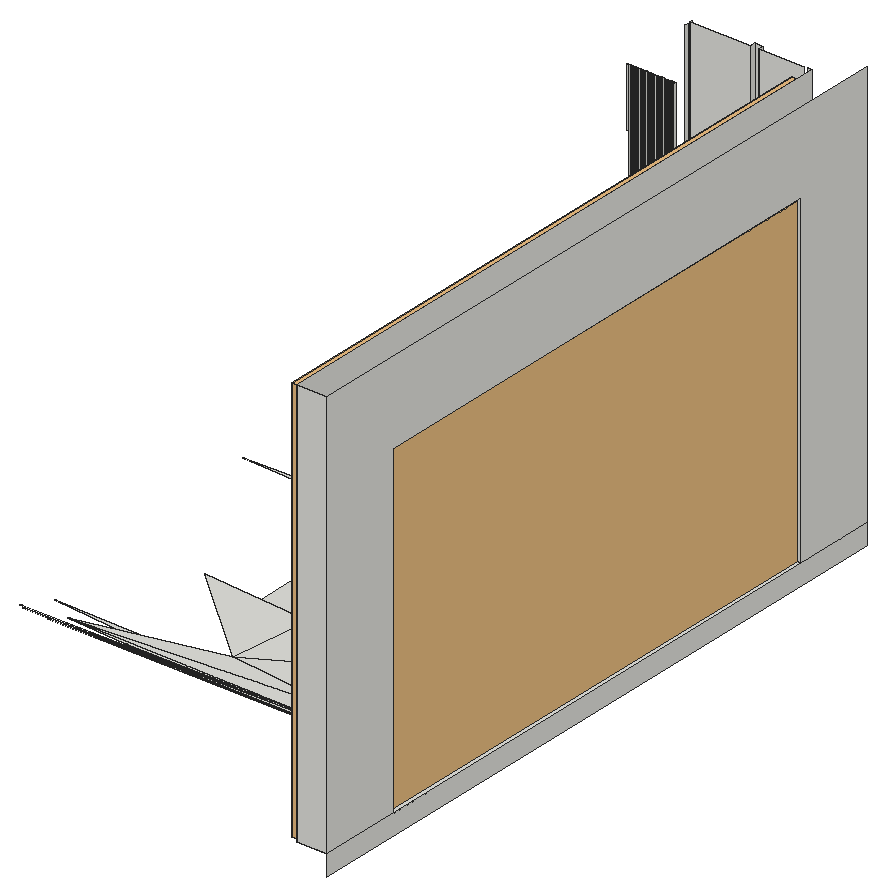
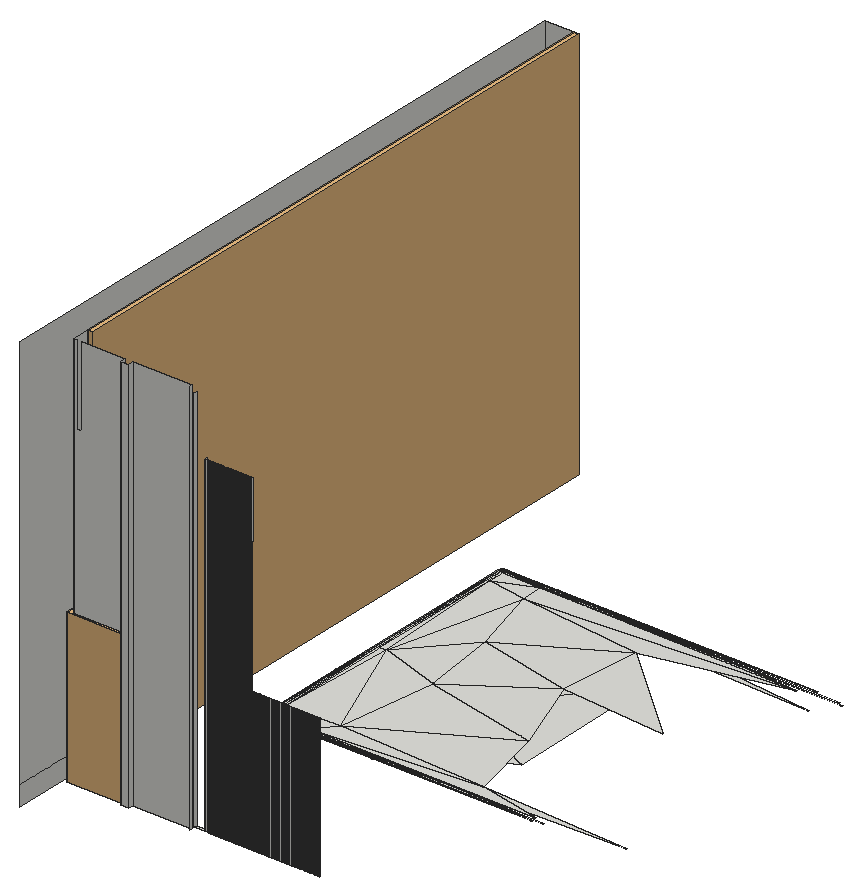
# SketchUp Ruby script. Lengths in inches.
U = 1.inch
M = Sketchup.active_model
def pt(a) = Geom::Point3d.new(a.map { |v| v * U })
def face(e, loops, mat)
  f = e.add_face(loops[0].map { |a| pt(a) })
  loops[1..].each { |l| e.add_face(l.map { |a| pt(a) }).erase! }
  f.material = f.back_material = mat if mat
  f
end
# faces: each face lists its corners as indices into pts; further lists are holes
def faces(e, pts, list, mat = nil) = list.each { |f| face(e, (f[0].is_a?(Array) ? f : [f]).map { |l| l.map { |i| pts[i] } }, mat) }
# xy, xz, yz: faces in a plane at the given z, y or x. An outline is a flat list of corners, or four numbers for a rectangle; further outlines are holes
def ring(l) = l.size == 4 ? [[l[0], l[1]], [l[2], l[1]], [l[2], l[3]], [l[0], l[3]]] : l.each_slice(2).to_a
def flat(e, list, mat, &to3) = list.each { |f| face(e, (f[0].is_a?(Array) ? f : [f]).map { |l| ring(l).map { |u, v| to3.(u, v) } }, mat) }
def xy(e, z, list, mat = nil) = flat(e, list, mat) { |x, y| [x, y, z] }
def xz(e, y, list, mat = nil) = flat(e, list, mat) { |x, z| [x, y, z] }
def yz(e, x, list, mat = nil) = flat(e, list, mat) { |y, z| [x, y, z] }
def lines(e, pts, list) = list.each { |a, b| e.add_line(pt(pts[a]), pt(pts[b])) }
# prism: a flat outline (further loops are holes) pulled along v
def prism(e, loops, v, mat = nil)
  f = face(e, loops, mat); d = Geom::Vector3d.new(v.map { |x| x * U })
  f.pushpull(f.normal.samedirection?(d) ? d.length : -d.length)
end
def box(e, o, s, mat = nil) = prism(e, [[o, [o[0] + s[0], o[1], o[2]], [o[0] + s[0], o[1] + s[1], o[2]], [o[0], o[1] + s[1], o[2]]]], [0, 0, s[2]], mat)
def at(x, y, z, deg = 0) = Geom::Transformation.translation(pt([x, y, z])) * Geom::Transformation.rotation(ORIGIN, Z_AXIS, deg.degrees)
def axes(o, x, y, z) = Geom::Transformation.new([*x, 0, *y, 0, *z, 0, *pt(o).to_a, 1])
def part(name) = M.definitions.add(name)
# library, detail: a bought-in or finely detailed component or shape, given as its bounding box
def library(name, o, s) = part(name).tap { |d| box(d.entities, o, s) }
def detail(e, o, s) = box(e.add_group.entities, o, s)
def put(e, d, t, mat = nil) = e.add_instance(d, t).tap { |i| i.material = mat if mat }
def group(e, t, mat = nil) = e.add_group.tap { |g| g.transformation = t; g.material = mat if mat }.entities
root = M.entities
c1 = library("Potted Plant 60-25",[-10.7,-10.47,0],[21.2,21.27,47.12])
c2 = library("Curtains 001",[-91.88,-6.87,0.16],[183.71,15.03,109.46])
c3 = library("Window 46-47",[-61.02,-2.17,0],[122.04,4.34,74.02])
xy(root,0,[[189,0,198,24],[189,24,198,174],[79.4375,45.79,129.55,46.18,156.43,45.79],[156.43,45.79,129.55,46.18,161.8,46.18],[156.43,45.79,161.8,46.18,172.9375,45.79],
  [172.9375,45.79,161.8,46.18,172.63,46.18],[172.9375,45.79,172.63,46.18,173.24,46.18],[172.9375,45.79,173.24,46.18,173.85,45.82],[173.85,45.82,173.24,46.18,173.85,46.18],[173.85,45.82,173.85,46.18,174.1875,45.84],
  [174.1875,45.84,173.85,46.18,174.21,46.18],[71.8,46.18,142.125,46.79,129.55,46.18],[129.55,46.18,142.125,46.79,161.8,46.18],[161.8,46.18,142.125,46.79,172.63,46.79],[161.8,46.18,172.63,46.79,172.63,46.18],
  [172.63,46.18,172.63,46.79,173.24,46.18],[173.24,46.18,172.63,46.79,173.24,46.79],[173.24,46.18,173.24,46.79,173.85,46.18],[173.85,46.18,173.24,46.79,173.85,46.79],[173.85,46.18,173.85,46.79,174.21,46.18],
  [174.21,46.18,173.85,46.79,174.25,47.09],[70.45,46.79,143.14,47.4,142.125,46.79],[142.125,46.79,143.14,47.4,172.63,46.79],[172.63,46.79,143.14,47.4,172.63,47.97],[172.63,46.79,172.63,47.97,173.24,47.4],
  [172.63,46.79,173.24,47.4,173.24,46.79],[173.24,46.79,173.24,47.4,173.85,46.79],[173.85,46.79,173.24,47.4,173.85,47.4],[173.85,46.79,173.85,47.4,174.25,47.09],[174.25,47.09,173.85,47.4,173.85,59.65],
  [174.25,47.09,173.85,59.65,174.25,74.37],[143.14,47.4,75.08,53.77,149.74,51.96],[143.14,47.4,149.74,51.96,172.63,47.97],[173.24,47.4,172.63,47.97,173.24,94.83],[173.24,47.4,173.24,94.83,173.85,59.65],
  [173.24,47.4,173.85,59.65,173.85,47.4],[172.63,47.97,149.74,51.96,169.97,85.51],[172.63,47.97,169.97,85.51,172.63,84.58],[172.63,47.97,172.63,84.58,173.24,94.83],[149.74,51.96,112.4,68.43,138.46,72.11],
  [149.74,51.96,138.46,72.11,169.97,85.51],[173.85,59.65,173.24,94.83,173.85,111.88],[173.85,59.65,173.85,111.88,174.25,74.37],[112.4,68.43,111.5,116.5625,139.8,102.6],[112.4,68.43,139.8,102.6,138.46,72.11],
  [138.46,72.11,139.8,102.6,158.95,87.44],[138.46,72.11,158.95,87.44,169.97,85.51],[174.25,74.37,173.85,111.88,174.25,122.24],[172.63,84.58,169.97,85.51,170.01,129.8],[172.63,84.58,170.01,129.8,172.63,133.19],
  [172.63,84.58,172.63,133.19,173.24,94.83],[169.97,85.51,139.65,129.14,170.01,129.8],[169.97,85.51,139.8,102.6,139.65,129.14],[169.97,85.51,158.95,87.44,139.8,102.6],[173.24,94.83,172.63,133.19,173.24,134.57],
  [173.24,94.83,173.24,134.57,173.85,111.88],[139.8,102.6,111.5,116.5625,139.65,129.14],[173.85,111.88,173.24,134.57,173.85,134.57],[173.85,111.88,173.85,134.57,174.25,122.24],[174.25,122.24,173.85,134.57,174.25,134.87],
  [139.65,129.14,67.21,132.46,139.03,134.57],[139.65,129.14,139.03,134.57,170.01,129.8],[170.01,129.8,139.03,134.57,172.63,134.57],[170.01,129.8,172.63,134.57,172.63,133.19],[172.63,133.19,172.63,134.57,173.24,134.57],
  [139.03,134.57,110.28,135.18,156.43,135.18],[139.03,134.57,156.43,135.18,172.63,134.57],[172.63,134.57,156.43,135.18,172.63,135.18],[172.63,134.57,172.63,135.18,173.24,134.57],[173.24,134.57,172.63,135.18,173.24,135.18],
  [173.24,134.57,173.24,135.18,173.85,134.57],[173.85,134.57,173.24,135.18,173.85,135.18],[173.85,134.57,173.85,135.18,174.25,134.87],[174.25,134.87,173.85,135.18,174.21,135.79],[110.28,135.18,92.94,135.79,145.92,135.79],
  [110.28,135.18,145.92,135.79,156.43,135.18],[156.43,135.18,145.92,135.79,168.42,135.79],[156.43,135.18,168.42,135.79,172.63,135.18],[172.63,135.18,168.42,135.79,172.63,135.79],[172.63,135.18,172.63,135.79,173.24,135.18],
  [173.24,135.18,172.63,135.79,173.24,135.79],[173.24,135.18,173.24,135.79,173.85,135.18],[173.85,135.18,173.24,135.79,173.85,135.79],[173.85,135.18,173.85,135.79,174.21,135.79],[92.94,135.79,140.64,136.17,145.92,135.79],
  [145.92,135.79,140.64,136.17,168.42,135.79],[168.42,135.79,140.64,136.17,172.63,136.17],[168.42,135.79,172.63,136.17,172.63,135.79],[172.63,135.79,172.63,136.17,173.24,135.79],[173.24,135.79,172.63,136.17,173.24,136.17],
  [173.24,135.79,173.24,136.17,173.85,136.14],[173.24,135.79,173.85,136.14,173.85,135.79],[173.85,135.79,173.85,136.14,174.21,135.79],[171.08,189,173.42,190.5]])
xy(root,0.23,[[157.71,45.79,158.28,46.18,96.94,46.18],[157.71,45.79,172.9375,45.79,158.28,46.18],[172.9375,45.79,172.63,46.18,158.28,46.18],[172.9375,45.79,173.24,46.18,172.63,46.18],[172.9375,45.79,173.85,45.82,173.24,46.18],
  [173.85,45.82,173.85,46.18,173.24,46.18],[173.85,45.82,174.21,46.18,173.85,46.18],[96.94,46.18,158.28,46.18,150.44,46.79],[158.28,46.18,172.63,46.79,150.44,46.79],[158.28,46.18,172.63,46.18,172.63,46.79],
  [172.63,46.18,173.24,46.18,173.24,46.79],[172.63,46.18,173.24,46.79,172.63,46.79],[173.24,46.18,173.85,46.18,173.85,46.79],[173.24,46.18,173.85,46.79,173.24,46.79],[173.85,46.18,174.21,46.18,173.85,46.79],
  [174.21,46.18,174.25,47.09,173.85,46.79],[150.44,46.79,161.16,47.4,101.08,47.4],[150.44,46.79,172.63,46.79,161.16,47.4],[172.63,46.79,172.63,47.4,161.16,47.4],[172.63,46.79,173.24,46.79,173.24,47.4],
  [172.63,46.79,173.24,47.4,172.63,47.4],[173.24,46.79,173.85,46.79,173.85,47.4],[173.24,46.79,173.85,47.4,173.24,47.4],[173.85,46.79,174.25,47.09,173.85,47.4],[174.25,47.09,173.85,61.21,173.85,47.4],
  [174.25,47.09,174.25,62.35,173.85,61.21],[101.08,47.4,161.16,47.4,82.99,48.58],[161.16,47.4,161,54.02,82.99,48.58],[161.16,47.4,172.63,52.46,161,54.02],[161.16,47.4,172.63,47.4,172.63,52.46],
  [172.63,47.4,173.24,47.4,172.63,52.46],[173.24,47.4,173.24,85.125,172.63,52.46],[173.24,47.4,173.85,47.4,173.85,61.21],[173.24,47.4,173.85,61.21,173.24,85.125],[82.99,48.58,161,54.02,124,57.84],
  [172.63,52.46,170.8,93.47,161,54.02],[172.63,52.46,172.63,93.73,170.8,93.47],[172.63,52.46,173.24,85.125,172.63,93.73],[161,54.02,155.14,75.83,124,57.84],[161,54.02,170.8,93.47,155.14,75.83],
  [124,57.84,126.68,81.95,94.82,84.31],[124,57.84,155.14,75.83,126.68,81.95],[173.85,61.21,173.85,111.56,173.24,85.125],[173.85,61.21,174.25,62.35,173.85,111.56],[174.25,62.35,174.25,108.12,173.85,111.56],
  [155.14,75.83,152.13,99.47,126.68,81.95],[155.14,75.83,170.8,93.47,152.13,99.47],[126.68,81.95,152.13,99.47,117.31,106.81],[173.24,85.125,172.63,129.16,172.63,93.73],[173.24,85.125,173.24,134.57,172.63,129.16],
  [173.24,85.125,173.85,111.56,173.24,134.57],[170.8,93.47,156.54,128.69,152.13,99.47],[170.8,93.47,172.63,129.16,156.54,128.69],[170.8,93.47,172.63,93.73,172.63,129.16],[152.13,99.47,156.54,128.69,117.31,106.81],
  [117.31,106.81,156.54,128.69,111.91,130.52],[174.25,108.12,174.25,134.87,173.85,111.56],[173.85,111.56,173.85,134.57,173.24,134.57],[173.85,111.56,174.25,134.87,173.85,134.57],[156.54,128.69,161.15,134.57,111.91,130.52],
  [156.54,128.69,172.63,129.16,161.15,134.57],[172.63,129.16,172.63,134.57,161.15,134.57],[172.63,129.16,173.24,134.57,172.63,134.57],[111.91,130.52,161.15,134.57,92.98,134.57],[92.98,134.57,161.15,134.57,121.1,135.18],
  [161.15,134.57,162.79,135.18,121.1,135.18],[161.15,134.57,172.63,134.57,162.79,135.18],[172.63,134.57,172.63,135.18,162.79,135.18],[172.63,134.57,173.24,134.57,173.24,135.18],[172.63,134.57,173.24,135.18,172.63,135.18],
  [173.24,134.57,173.85,134.57,173.85,135.18],[173.24,134.57,173.85,135.18,173.24,135.18],[173.85,134.57,174.25,134.87,173.85,135.18],[174.25,134.87,174.21,135.79,173.85,135.18],[121.1,135.18,134.45,135.79,89.4,135.79],
  [121.1,135.18,162.6875,135.78,134.45,135.79],[121.1,135.18,162.79,135.18,162.6875,135.78],[162.79,135.18,172.63,135.79,162.6875,135.78],[162.79,135.18,172.63,135.18,172.63,135.79],[172.63,135.18,173.24,135.18,173.24,135.79],
  [172.63,135.18,173.24,135.79,172.63,135.79],[173.24,135.18,173.85,135.18,173.85,135.79],[173.24,135.18,173.85,135.79,173.24,135.79],[173.85,135.18,174.21,135.79,173.85,135.79],[162.6875,135.78,156.13,136.17,134.45,135.79],
  [162.6875,135.78,172.9375,136.17,156.13,136.17],[162.6875,135.78,172.63,135.79,172.9375,136.17],[134.45,135.79,156.13,136.17,115.29,136.17],[172.63,135.79,173.24,135.79,172.9375,136.17],[173.24,135.79,173.85,136.14,172.9375,136.17],
  [173.24,135.79,173.85,135.79,173.85,136.14],[173.85,135.79,174.1875,136.125,173.85,136.14],[173.85,135.79,174.21,135.79,174.1875,136.125]])
xy(root,1.3,[[148.625,189,151.87,189.875],[134.28,189.625,134.875,189.875],[124.28,189.75,124.875,189.875],[125.28,189.75,125.875,189.875],[126.28,189.75,126.875,189.875],
  [127.28,189.75,127.875,189.875],[128.28,189.75,128.875,189.875],[129.28,189.75,129.875,189.875],[130.28,189.75,130.875,189.875],[131.28,189.75,131.875,189.875],
  [132.28,189.75,132.875,189.875],[133.28,189.75,133.875,189.875],[135.28,189.75,135.875,189.875],[136.28,189.75,136.875,189.875],[137.28,189.75,137.875,189.875],
  [138.28,189.75,138.875,189.875],[139.28,189.75,139.875,189.875],[140.28,189.75,140.875,189.875],[141.28,189.75,141.875,189.875],[142.28,189.75,142.875,189.875],
  [143.28,189.75,143.875,189.875],[144.28,189.75,144.875,189.875],[145.28,189.75,145.875,189.875],[146.28,189.75,146.875,189.875],[147.28,189.75,147.875,189.875],
  [114.28,189.8125,114.875,189.875],[115.28,189.8125,115.875,189.875],[116.28,189.8125,116.875,189.875],[117.28,189.8125,117.875,189.875],[118.28,189.8125,118.875,189.875],
  [119.28,189.8125,119.875,189.875],[120.28,189.8125,120.875,189.875],[121.28,189.8125,121.875,189.875],[122.28,189.8125,122.875,189.875],[123.28,189.8125,123.875,189.875]])
xz(root,0,[[189,0,198,120]])
xz(root,24,[[189,0,198,96]])
xz(root,45.79,[[156.43,0,157.71,0.23,78.85,0.23],[156.43,0,172.9375,0,157.71,0.23],[172.9375,0,172.9375,0.23,157.71,0.23]])
xz(root,136.17,[[140.64,0,115.29,0.23,156.13,0.23],[140.64,0,156.13,0.23,172.63,0],[172.63,0,156.13,0.23,172.9375,0.23],[172.63,0,172.9375,0.23,173.24,0]])
xz(root,174,[[189,0,198,96]])
xz(root,189,[[153.17,0,171.08,120],[173.42,0,189,0,189,120,187.95,120,187.95,96,186.625,96,186.625,120,173.42,120]])
xz(root,189.625,[[134.28,1.3,134.875,1.3,134.875,101.92,134.28,101.92,134.28,84.67,134.75,84.67,134.75,44.04,134.28,44.04]])
xz(root,189.75,[[124.28,1.3,124.875,44.04],[125.28,1.3,125.875,44.04],[126.28,1.3,126.875,44.04],[127.28,1.3,127.875,44.04],[128.28,1.3,128.875,44.04],
  [129.28,1.3,129.875,44.04],[130.28,1.3,130.875,44.04],[131.28,1.3,131.875,44.04],[132.28,1.3,132.875,44.04],[133.28,1.3,133.875,44.04],
  [135.28,1.3,135.875,101.92],[136.28,1.3,136.875,101.92],[137.28,1.3,137.875,101.92],[138.28,1.3,138.875,101.92],[139.28,1.3,139.875,101.92],
  [140.28,1.3,140.875,101.92],[141.28,1.3,141.875,101.92],[142.28,1.3,142.875,101.92],[143.28,1.3,143.875,101.92],[144.28,1.3,144.875,101.92],
  [145.28,1.3,145.875,101.92],[146.28,1.3,146.875,101.92],[147.28,1.3,147.875,101.92]])
xz(root,189.8125,[[114.28,1.3,114.875,44.04],[115.28,1.3,115.875,44.04],[116.28,1.3,116.875,44.04],[117.28,1.3,117.875,44.04],[118.28,1.3,118.875,44.04],
  [119.28,1.3,119.875,44.04],[120.28,1.3,120.875,44.04],[121.28,1.3,121.875,44.04],[122.28,1.3,122.875,44.04],[123.28,1.3,123.875,44.04]])
xz(root,189.875,[[113.875,1.3,114.28,44.04],[114.875,1.3,115.28,44.04],[115.875,1.3,116.28,44.04],[116.875,1.3,117.28,44.04],[117.875,1.3,118.28,44.04],
  [118.875,1.3,119.28,44.04],[119.875,1.3,120.28,44.04],[120.875,1.3,121.28,44.04],[121.875,1.3,122.28,44.04],[122.875,1.3,123.28,44.04],
  [123.875,1.3,124.28,44.04],[124.875,1.3,125.28,44.04],[125.875,1.3,126.28,44.04],[126.875,1.3,127.28,44.04],[127.875,1.3,128.28,44.04],
  [128.875,1.3,129.28,44.04],[129.875,1.3,130.28,44.04],[130.875,1.3,131.28,44.04],[131.28,1.3,131.875,44.04],[131.875,1.3,132.28,44.04],
  [132.28,1.3,132.875,44.04],[132.875,1.3,133.28,44.04],[133.28,1.3,133.875,44.04],[133.875,1.3,134.28,44.04],[134.28,1.3,134.28,44.04,134.75,44.04,134.75,84.67,134.28,84.67,134.28,101.92,134.875,101.92,134.875,1.3],
  [134.875,1.3,135.28,101.92],[135.28,1.3,135.875,101.92],[135.875,1.3,136.28,101.92],[136.28,1.3,136.875,101.92],[136.875,1.3,137.28,101.92],
  [137.28,1.3,137.875,101.92],[137.875,1.3,138.28,101.92],[138.28,1.3,138.875,101.92],[138.875,1.3,139.28,101.92],[139.28,1.3,139.875,101.92],
  [139.875,1.3,140.28,101.92],[140.28,1.3,140.875,101.92],[140.875,1.3,141.28,101.92],[141.28,1.3,141.875,101.92],[141.875,1.3,142.28,101.92],
  [142.28,1.3,142.875,101.92],[142.875,1.3,143.28,101.92],[143.28,1.3,143.875,101.92],[143.875,1.3,144.28,101.92],[144.28,1.3,144.875,101.92],
  [144.875,1.3,145.28,101.92],[145.28,1.3,145.875,101.92],[145.875,1.3,146.28,101.92],[146.28,1.3,146.875,101.92],[146.875,1.3,147.28,101.92],
  [147.28,1.3,147.875,101.92],[147.875,1.3,148.625,101.92]])
xz(root,190.5,[[171.08,0,173.42,120]])
yz(root,113.875,[[189.8125,1.3,189.875,44.04]])
yz(root,114.28,[[189.8125,1.3,189.875,44.04]])
yz(root,114.875,[[189.8125,1.3,189.875,44.04]])
yz(root,115.28,[[189.8125,1.3,189.875,44.04]])
yz(root,115.875,[[189.8125,1.3,189.875,44.04]])
yz(root,116.28,[[189.8125,1.3,189.875,44.04]])
yz(root,116.875,[[189.8125,1.3,189.875,44.04]])
yz(root,117.28,[[189.8125,1.3,189.875,44.04]])
yz(root,117.875,[[189.8125,1.3,189.875,44.04]])
yz(root,118.28,[[189.8125,1.3,189.875,44.04]])
yz(root,118.875,[[189.8125,1.3,189.875,44.04]])
yz(root,119.28,[[189.8125,1.3,189.875,44.04]])
yz(root,119.875,[[189.8125,1.3,189.875,44.04]])
yz(root,120.28,[[189.8125,1.3,189.875,44.04]])
yz(root,120.875,[[189.8125,1.3,189.875,44.04]])
yz(root,121.28,[[189.8125,1.3,189.875,44.04]])
yz(root,121.875,[[189.8125,1.3,189.875,44.04]])
yz(root,122.28,[[189.8125,1.3,189.875,44.04]])
yz(root,122.875,[[189.8125,1.3,189.875,44.04]])
yz(root,123.28,[[189.8125,1.3,189.875,44.04]])
yz(root,123.875,[[189.8125,1.3,189.875,44.04]])
yz(root,124.28,[[189.75,1.3,189.875,44.04]])
yz(root,124.875,[[189.75,1.3,189.875,44.04]])
yz(root,125.28,[[189.75,1.3,189.875,44.04]])
yz(root,125.875,[[189.75,1.3,189.875,44.04]])
yz(root,126.28,[[189.75,1.3,189.875,44.04]])
yz(root,126.875,[[189.75,1.3,189.875,44.04]])
yz(root,127.28,[[189.75,1.3,189.875,44.04]])
yz(root,127.875,[[189.75,1.3,189.875,44.04]])
yz(root,128.28,[[189.75,1.3,189.875,44.04]])
yz(root,128.875,[[189.75,1.3,189.875,44.04]])
yz(root,129.28,[[189.75,1.3,189.875,44.04]])
yz(root,129.875,[[189.75,1.3,189.875,44.04]])
yz(root,130.28,[[189.75,1.3,189.875,44.04]])
yz(root,130.875,[[189.75,1.3,189.875,44.04]])
yz(root,131.28,[[189.75,1.3,189.875,44.04]])
yz(root,131.875,[[189.75,1.3,189.875,44.04]])
yz(root,132.28,[[189.75,1.3,189.875,44.04]])
yz(root,132.875,[[189.75,1.3,189.875,44.04]])
yz(root,133.28,[[189.75,1.3,189.875,44.04]])
yz(root,133.875,[[189.75,1.3,189.875,44.04]])
yz(root,134.28,[[189.625,1.3,189.875,44.04]])
yz(root,134.875,[[189.625,1.3,189.875,101.92]])
yz(root,135.28,[[189.75,1.3,189.875,101.92]])
yz(root,135.875,[[189.75,1.3,189.875,101.92]])
yz(root,136.28,[[189.75,1.3,189.875,101.92]])
yz(root,136.875,[[189.75,1.3,189.875,101.92]])
yz(root,137.28,[[189.75,1.3,189.875,101.92]])
yz(root,137.875,[[189.75,1.3,189.875,101.92]])
yz(root,138.28,[[189.75,1.3,189.875,101.92]])
yz(root,138.875,[[189.75,1.3,189.875,101.92]])
yz(root,139.28,[[189.75,1.3,189.875,101.92]])
yz(root,139.875,[[189.75,1.3,189.875,101.92]])
yz(root,140.28,[[189.75,1.3,189.875,101.92]])
yz(root,140.875,[[189.75,1.3,189.875,101.92]])
yz(root,141.28,[[189.75,1.3,189.875,101.92]])
yz(root,141.875,[[189.75,1.3,189.875,101.92]])
yz(root,142.28,[[189.75,1.3,189.875,101.92]])
yz(root,142.875,[[189.75,1.3,189.875,101.92]])
yz(root,143.28,[[189.75,1.3,189.875,101.92]])
yz(root,143.875,[[189.75,1.3,189.875,101.92]])
yz(root,144.28,[[189.75,1.3,189.875,101.92]])
yz(root,144.875,[[189.75,1.3,189.875,101.92]])
yz(root,145.28,[[189.75,1.3,189.875,101.92]])
yz(root,145.875,[[189.75,1.3,189.875,101.92]])
yz(root,146.28,[[189.75,1.3,189.875,101.92]])
yz(root,146.875,[[189.75,1.3,189.875,101.92]])
yz(root,147.28,[[189.75,1.3,189.875,101.92]])
yz(root,147.875,[[189.75,1.3,189.875,101.92]])
yz(root,148.625,[[189,1.3,189.875,101.92]])
yz(root,151.87,[[189,1.3,189.875,118.7]])
yz(root,153.17,[[189,0,189.875,120]])
yz(root,171.08,[[189,0,190.5,120]])
yz(root,173.42,[[189,0,190.5,120]])
yz(root,174.25,[[47.09,0,62.35,0.23,47.09,0.23],[47.09,0,74.37,0,62.35,0.23],[74.37,0,108.12,0.23,62.35,0.23],[74.37,0,122.24,0,108.12,0.23],[122.24,0,134.87,0.23,108.12,0.23],
  [122.24,0,134.87,0,134.87,0.23]])
yz(root,189,[[0,0,0,120,189,120,189,0,174,0,174,96,24,96,24,0]])
yz(root,198,[[0,-6,198,0],[0,0,24,0,24,96,174,96,174,0,198,0,198,120,0,120]])
p = [[173.85,45.82,0.23],[172.9375,45.79,0.23],[172.9375,45.79,0],[173.85,45.82,0],[174.1875,45.84,0],[174.21,46.18,0.23],
  [174.21,46.18,0],[174.25,47.09,0.23],[174.25,47.09,0],[174.25,134.87,0],[174.21,135.79,0],[174.21,135.79,0.23],
  [174.25,134.87,0.23],[173.85,136.14,0],[174.1875,136.125,0.23],[173.24,136.17,0],[172.9375,136.17,0.23],[173.85,136.14,0.23]]
faces(root,p,[[0,1,2],[2,3,0],[0,3,4],[0,4,5],[4,6,5],[7,5,6],[6,8,7],[9,10,11],
  [11,12,9],[13,14,10],[11,10,14],[15,16,17],[17,13,15],[14,13,17]])
put(root,c1,axes([182.41,179.6,0],[0.7695,0,0],[0,0.95,0],[0,0,0.97232]))
put(root,c2,axes([188.33,91.88,0.52],[0,1,0],[-0.0972,0,0],[0,0,1.09]))
put(root,c3,axes([194.6,98.89,0],[0,1.22717,0],[-1,0,0],[0,0,1.28]))
